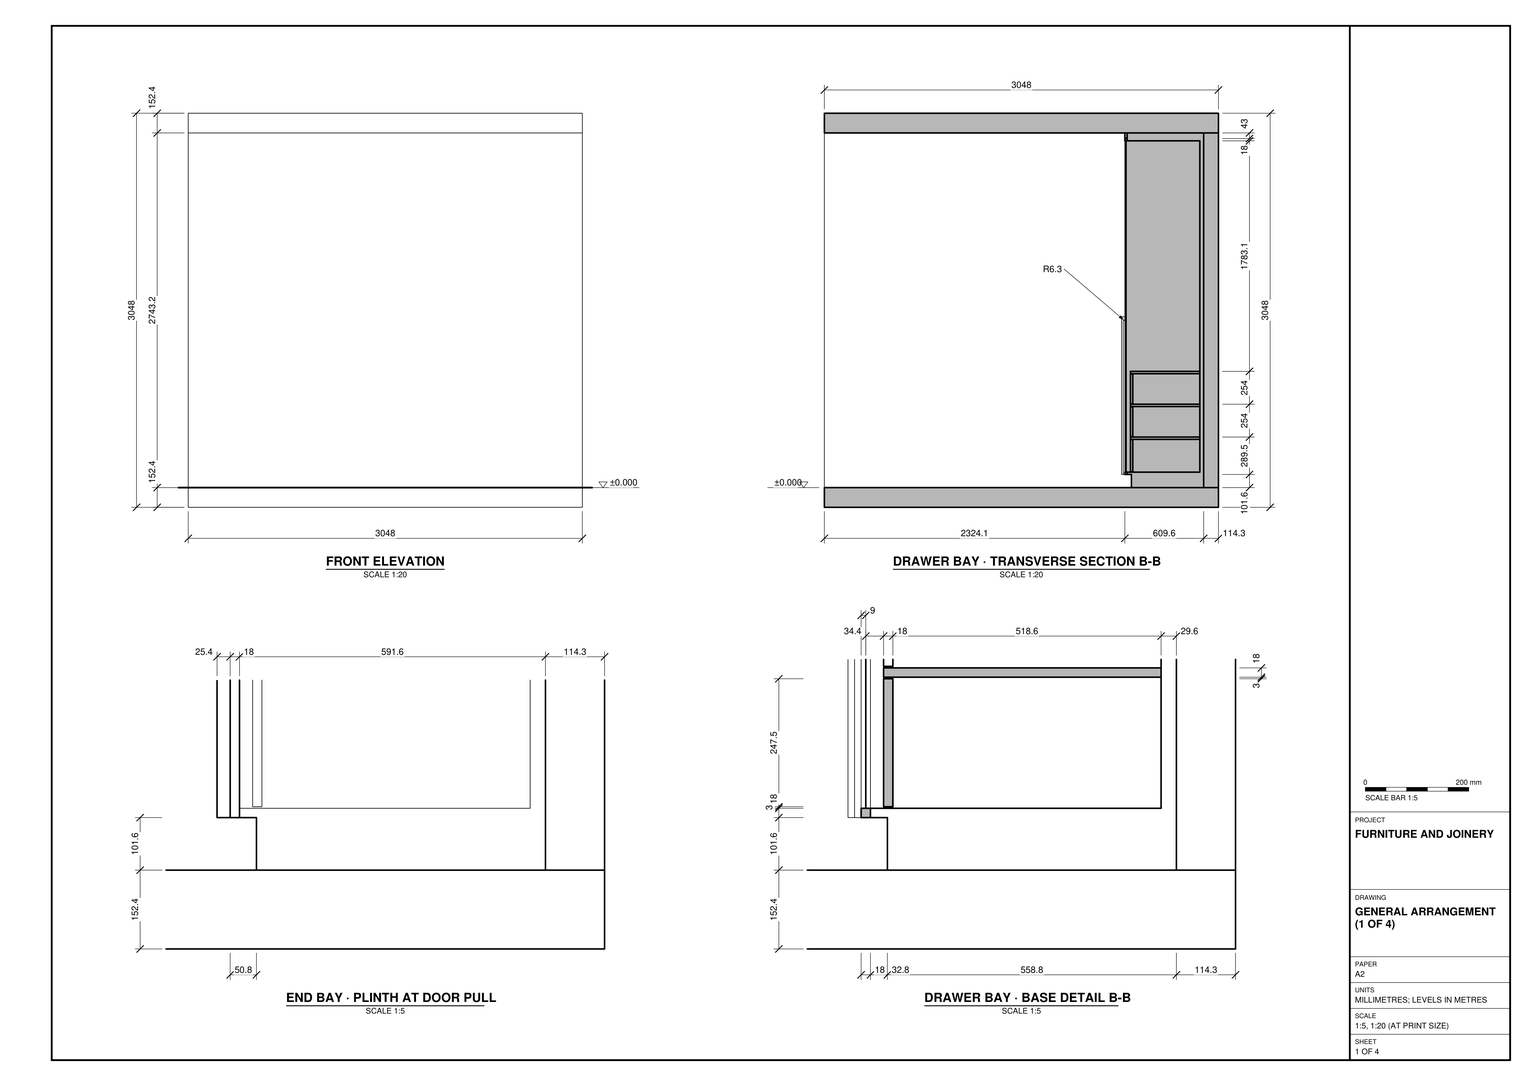
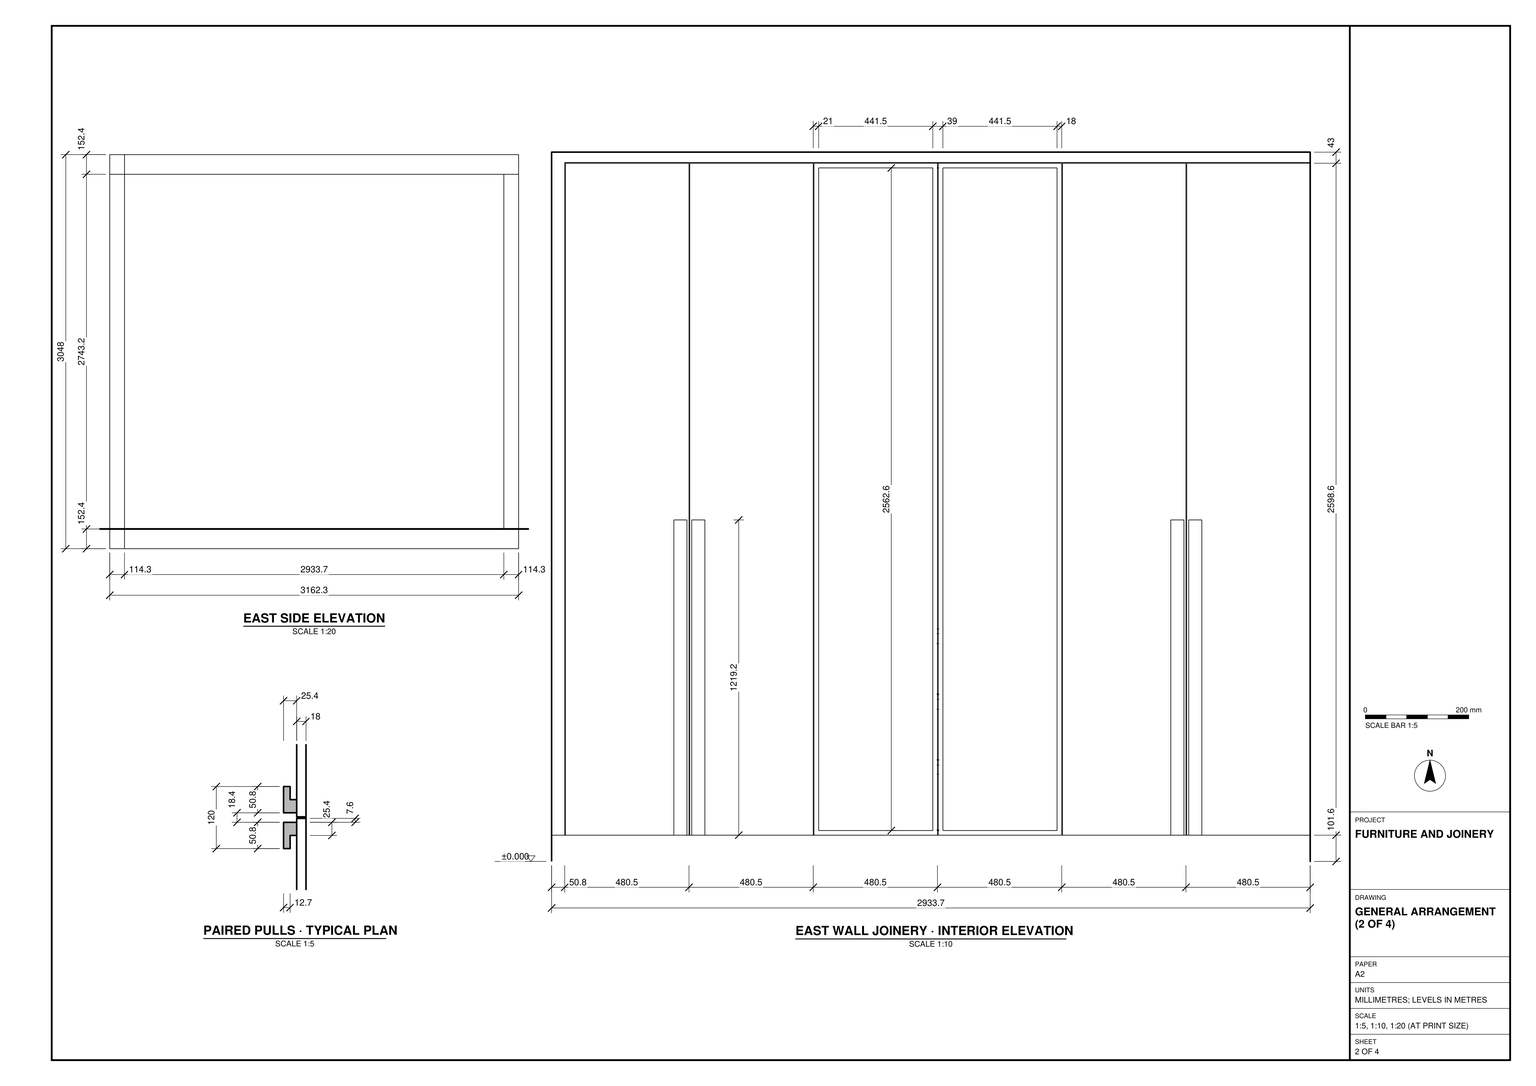
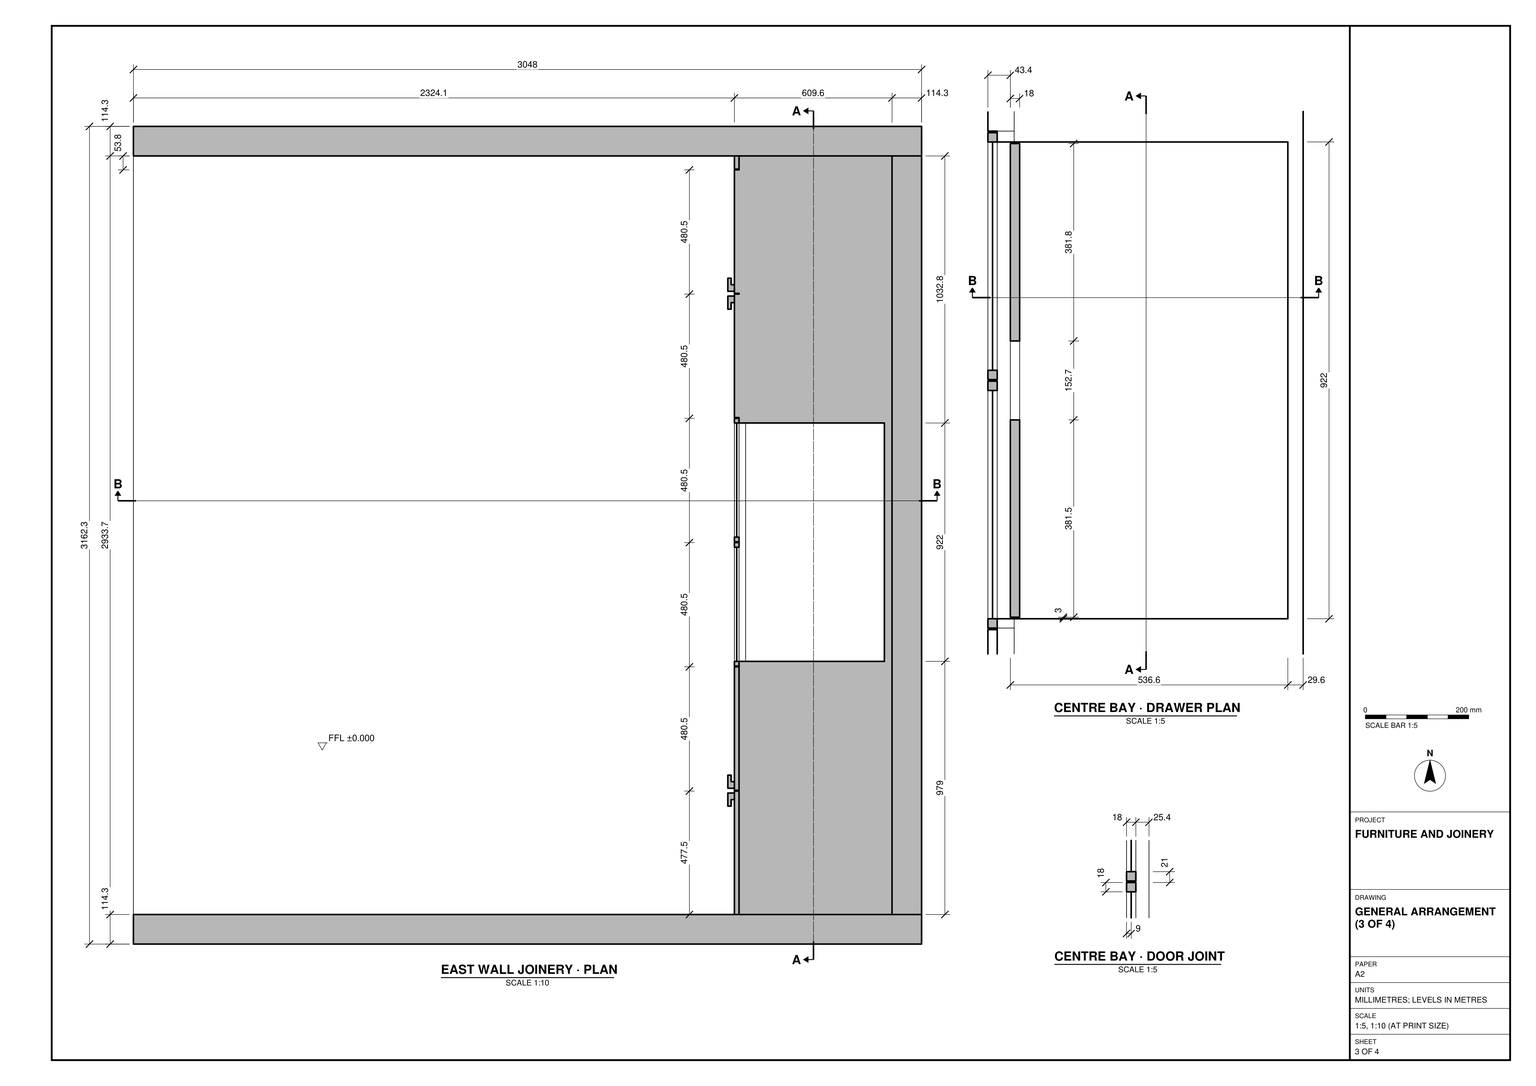
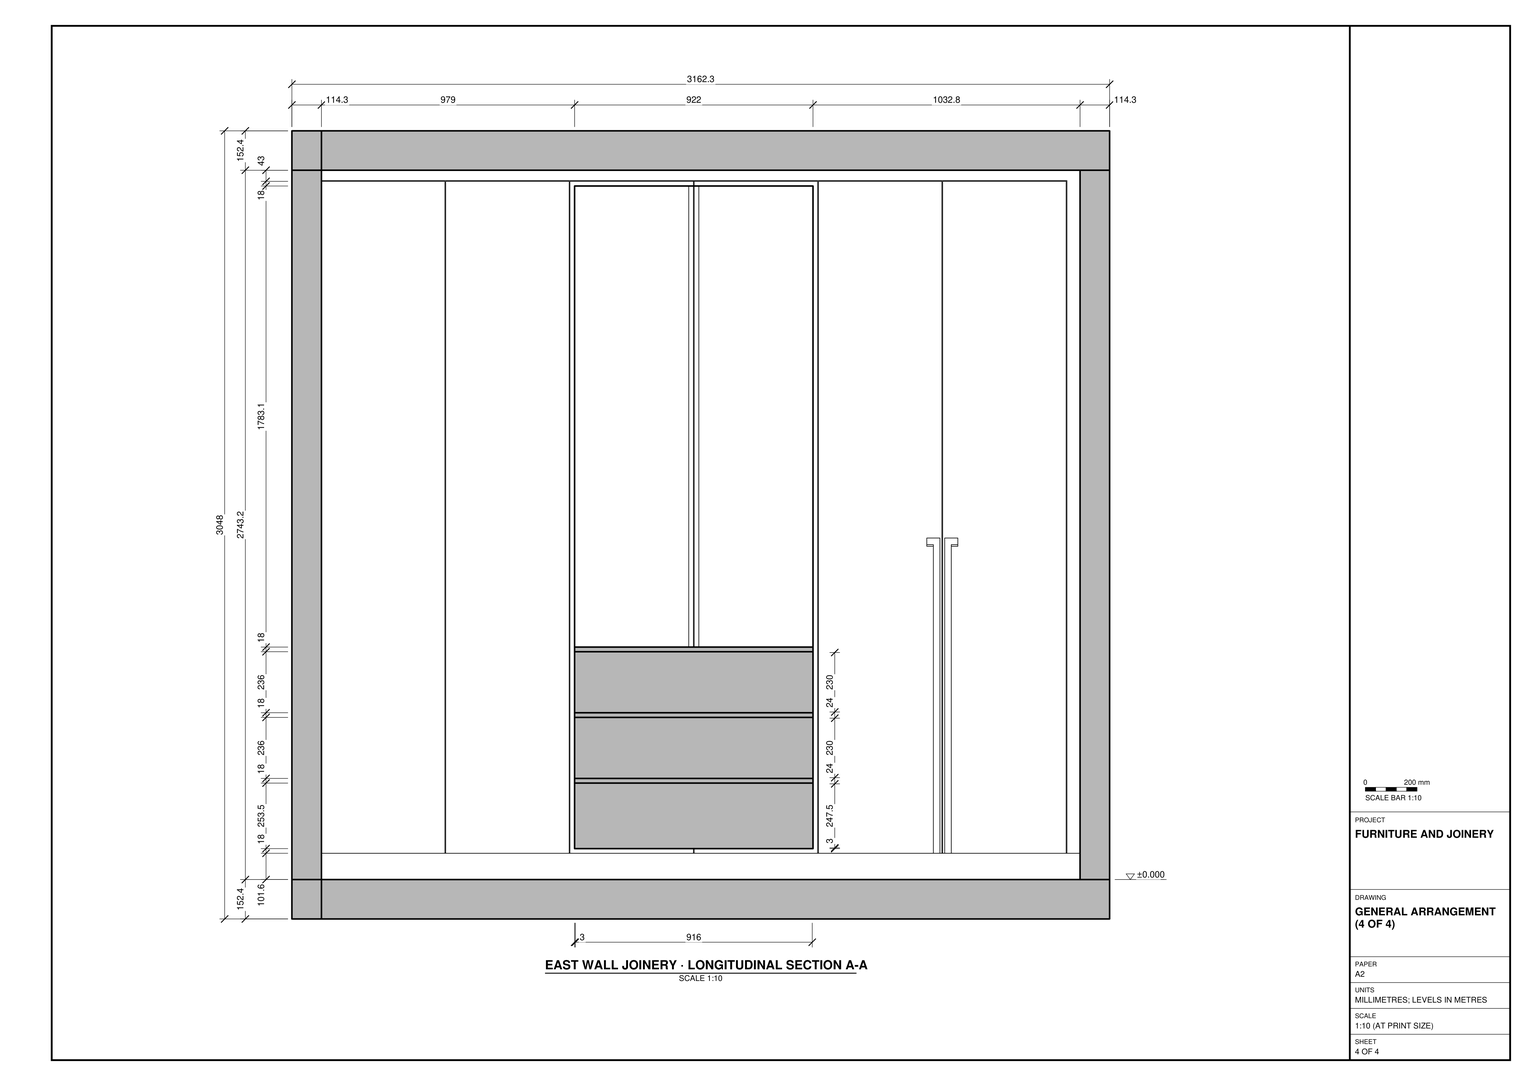
Work in millimetres in SketchUp from task_files/diagram_01.pdf. Model the full-height wardrobe along the east wall, together with the shell shown in plan and section. The overall extents are 3048 mm along X, 3162.3 mm along Y and 3048 mm vertically. Set the finished floor at the single storey level of 0 mm. Use the top of the floor slab, not its underside, as this datum. Model the floor and ceiling slabs and the east wall with its two return walls, leaving the opposite side open as drawn.

Fit the wardrobe between the return walls. Follow the interior elevation for the six tall fronts: the middle pair has narrow frames around inset panels, while the outer pairs have long vertical pulls at their meeting edges. Use the sections to set the cabinet depth, recess the plinth beneath the fronts and fit the narrow strip above them. Model the drawer stack low in the centre bay, leaving the space above it clear.

Keep the walls and slabs separate from one another and from the joinery. Organise the wardrobe and its distinct parts as groups or components, using components for repeated parts. Any decor or loose items may be suitable library components. Save one SketchUp model as output_files/east_wall_wardrobe_and_its_enclosing_shell.skp.

# SketchUp Ruby script. Lengths in millimetres.
U = 1.mm
M = Sketchup.active_model
def pt(a) = Geom::Point3d.new(a.map { |v| v * U })
def face(e, loops, mat)
  f = e.add_face(loops[0].map { |a| pt(a) })
  loops[1..].each { |l| e.add_face(l.map { |a| pt(a) }).erase! }
  f.material = f.back_material = mat if mat
  f
end
# faces: each face lists its corners as indices into pts; further lists are holes
def faces(e, pts, list, mat = nil) = list.each { |f| face(e, (f[0].is_a?(Array) ? f : [f]).map { |l| l.map { |i| pts[i] } }, mat) }
# xy, xz, yz: faces in a plane at the given z, y or x. An outline is a flat list of corners, or four numbers for a rectangle; further outlines are holes
def ring(l) = l.size == 4 ? [[l[0], l[1]], [l[2], l[1]], [l[2], l[3]], [l[0], l[3]]] : l.each_slice(2).to_a
def flat(e, list, mat, &to3) = list.each { |f| face(e, (f[0].is_a?(Array) ? f : [f]).map { |l| ring(l).map { |u, v| to3.(u, v) } }, mat) }
def xy(e, z, list, mat = nil) = flat(e, list, mat) { |x, y| [x, y, z] }
def xz(e, y, list, mat = nil) = flat(e, list, mat) { |x, z| [x, y, z] }
def yz(e, x, list, mat = nil) = flat(e, list, mat) { |y, z| [x, y, z] }
def lines(e, pts, list) = list.each { |a, b| e.add_line(pt(pts[a]), pt(pts[b])) }
# prism: a flat outline (further loops are holes) pulled along v
def prism(e, loops, v, mat = nil)
  f = face(e, loops, mat); d = Geom::Vector3d.new(v.map { |x| x * U })
  f.pushpull(f.normal.samedirection?(d) ? d.length : -d.length)
end
def box(e, o, s, mat = nil) = prism(e, [[o, [o[0] + s[0], o[1], o[2]], [o[0] + s[0], o[1] + s[1], o[2]], [o[0], o[1] + s[1], o[2]]]], [0, 0, s[2]], mat)
def at(x, y, z, deg = 0) = Geom::Transformation.translation(pt([x, y, z])) * Geom::Transformation.rotation(ORIGIN, Z_AXIS, deg.degrees)
def axes(o, x, y, z) = Geom::Transformation.new([*x, 0, *y, 0, *z, 0, *pt(o).to_a, 1])
def part(name) = M.definitions.add(name)
# library, detail: a bought-in or finely detailed component or shape, given as its bounding box
def library(name, o, s) = part(name).tap { |d| box(d.entities, o, s) }
def detail(e, o, s) = box(e.add_group.entities, o, s)
def put(e, d, t, mat = nil) = e.add_instance(d, t).tap { |i| i.material = mat if mat }
def group(e, t, mat = nil) = e.add_group.tap { |g| g.transformation = t; g.material = mat if mat }.entities
root = M.entities
M.materials.add("Tafisa-Mer-Calme-or-Calm-Sea-PM772-4K").color = [42, 58, 71]
M.materials.add("Tafisa-Rosee-du-Matin-or-Morning-Dew-PM763-4K").color = [198, 195, 187]
M.materials.add("[Color M09]").color = [0, 0, 0]
M.materials.add("[Translucent Glass Gray]").color = [128, 128, 128]
M.materials["[Translucent Glass Gray]"].alpha = 0.5
c1 = part("Group\#1")
xy(c1.entities,0,[[0,-114.3,3048,0],[0,0,3048,3048]])
xy(c1.entities,152.4,[[0,-114.3,3048,0],[0,0,3048,3048]])
xz(c1.entities,-114.3,[[0,0,3048,152.4]])
xz(c1.entities,0,[[0,0,3048,152.4]])
xz(c1.entities,3048,[[0,0,3048,152.4]])
yz(c1.entities,0,[[-114.3,0,0,152.4],[0,0,3048,152.4]])
yz(c1.entities,3048,[[-114.3,0,0,152.4],[0,0,3048,152.4]])
c2 = part("Group\#2")
box(c2.entities,[0,0,0],[3048,114.3,2743.2])
c3 = part("Group\#5")
box(c3.entities,[25.4,0,-18],[536.6,922,18])
c4 = part("Group\#9")
xy(c4.entities,0,[[0,0,0,50.8,25.4,50.8,25.4,25.4,12.7,25.4,12.7,0]])
xy(c4.entities,1219.2,[[0,0,25.4,50.8]])
xz(c4.entities,0,[[0,0,12.7,0,12.7,1187.2,12.9,1188.8,13.6,1190.4,14.6,1191.7,15.9,1192.7,17.4,1193.3,19,1193.6,20.7,1193.3,22.2,1192.7,23.5,1191.7,24.5,1190.4,25.2,1188.8,25.4,1187.2,25.4,1219.2,0,1219.2]])
xz(c4.entities,25.4,[[12.7,0,25.4,0,25.4,1187.2,25.2,1188.8,24.5,1190.4,23.5,1191.7,22.2,1192.7,20.7,1193.3,19,1193.6,17.4,1193.3,15.9,1192.7,14.6,1191.7,13.6,1190.4,12.9,1188.8,12.7,1187.2]])
xz(c4.entities,50.8,[[0,0,25.4,1219.2]])
yz(c4.entities,0,[[0,0,50.8,1219.2]])
yz(c4.entities,12.7,[[0,0,25.4,1187.2]])
yz(c4.entities,25.4,[[25.4,0,50.8,0,50.8,1219.2,0,1219.2,0,1187.2,25.4,1187.2]])
p = [[12.9,0,1188.8],[12.7,0,1187.2],[12.7,25.4,1187.2],[12.9,25.4,1188.8],[25.4,0,1187.2],[25.2,0,1188.8],
  [25.2,25.4,1188.8],[25.4,25.4,1187.2],[13.6,0,1190.4],[13.6,25.4,1190.4],[24.5,0,1190.4],[24.5,25.4,1190.4],
  [14.6,0,1191.7],[14.6,25.4,1191.7],[23.5,0,1191.7],[23.5,25.4,1191.7],[15.9,0,1192.7],[15.9,25.4,1192.7],
  [22.2,0,1192.7],[22.2,25.4,1192.7],[17.4,0,1193.3],[17.4,25.4,1193.3],[20.7,0,1193.3],[20.7,25.4,1193.3],
  [19,0,1193.6],[19,25.4,1193.6]]
faces(c4.entities,p,[[0,1,2,3],[4,5,6,7],[8,0,3,9],[5,10,11,6],[12,8,9,13],[10,14,15,11],[16,12,13,17],[14,18,19,15],
  [20,16,17,21],[18,22,23,19],[24,20,21,25],[22,24,25,23]])
yz(root,2333.1,[[1573.8,272,2015.2,2834.6]],"[Translucent Glass Gray]")
put(root,c1,at(0,114.3,0))
g1 = group(root,at(2933.7,114.3,152.4))
box(g1,[0,0,0],[114.3,2933.7,2743.2])
put(root,c2,at(0,3048,152.4))
g2 = group(root,at(2324.1,114.3,152.4),"Tafisa-Mer-Calme-or-Calm-Sea-PM772-4K")
xy(g2,0,[[50.8,0,609.6,2933.7]])
xy(g2,101.6,[[0,0,18,477.5],[18,0,50.8,961],[0,480.5,18,958],[18,961,50.8,1921.9],[0,1921.9,0,2399.4,18,2399.4,18,2402.4,0,2402.4,0,2879.9,18,2879.9,18,2882.9,50.8,2882.9,50.8,1921.9],
  [0,2882.9,18,2933.7],[18,2882.9,50.8,2933.7]])
xy(g2,101.6,[[0,961,18,1438.4],[0,1441.4,18,1918.9]],"[Color M09]")
xy(g2,119.6,[[18,979,580,1900.9]],"Tafisa-Rosee-du-Matin-or-Morning-Dew-PM763-4K")
xy(g2,119.6,[[0,979,9,1420.4],[9,979,18,1420.4],[0,1459.4,18,1900.9]],"[Color M09]")
xy(g2,2682.2,[[18,979,580,1900.9]],"Tafisa-Rosee-du-Matin-or-Morning-Dew-PM763-4K")
xy(g2,2682.2,[[0,979,9,1420.4],[9,979,18,1420.4],[0,1459.4,18,1900.9]],"[Color M09]")
xy(g2,2700.2,[[0,0,18,477.5],[0,480.5,18,958],[0,1921.9,18,2399.4],[0,2402.4,18,2879.9]])
xy(g2,2700.2,[[0,961,18,1438.5],[0,1441.5,18,1918.9]],"[Color M09]")
xy(g2,2703.2,[[0,0,18,2882.9]])
xy(g2,2743.2,[[0,0,18,2933.7],[18,0,609.6,2933.7]])
xz(g2,0,[[50.8,0,609.6,0,609.6,2743.2,18,2743.2,18,101.6,50.8,101.6],[0,101.6,18,2700.2],[0,2703.2,18,2743.2]])
xz(g2,477.5,[[0,101.6,18,2700.2]])
xz(g2,480.5,[[0,101.6,18,2700.2]])
xz(g2,958,[[0,101.6,18,2700.2]])
xz(g2,961,[[0,101.6,18,2700.2]])
xz(g2,979,[[18,119.6,580,2682.2]],"Tafisa-Rosee-du-Matin-or-Morning-Dew-PM763-4K")
xz(g2,979,[[0,119.6,9,2682.2],[9,119.6,18,2682.2]],"[Color M09]")
xz(g2,1420.4,[[0,119.6,9,2682.2],[9,119.6,18,2682.2]],"[Color M09]")
xz(g2,1459.4,[[0,119.6,18,2682.2]],"[Color M09]")
xz(g2,1900.9,[[18,119.6,580,2682.2]],"Tafisa-Rosee-du-Matin-or-Morning-Dew-PM763-4K")
xz(g2,1900.9,[[0,119.6,18,2682.2]],"[Color M09]")
xz(g2,1918.9,[[0,101.6,18,2700.2]],"[Color M09]")
xz(g2,1921.9,[[0,101.6,18,2700.2]])
xz(g2,2399.4,[[0,101.6,18,2700.2]])
xz(g2,2402.4,[[0,101.6,18,2700.2]])
xz(g2,2879.9,[[0,101.6,18,2700.2]])
xz(g2,2882.9,[[0,101.6,18,2703.2]])
xz(g2,2933.7,[[50.8,0,50.8,101.6,18,101.6,18,2743.2,609.6,2743.2,609.6,0],[0,101.6,18,2743.2]])
yz(g2,0,[[0,101.6,477.5,2700.2],[2882.9,101.6,2882.9,2703.2,0,2703.2,0,2743.2,2933.7,2743.2,2933.7,101.6],[480.5,101.6,958,2700.2],[1921.9,101.6,2399.4,2700.2],[2402.4,101.6,2879.9,2700.2]])
yz(g2,0,[[[961,101.6,961,2700.2,1438.5,2700.2,1438.4,101.6],[979,119.6,1420.4,2682.2]],[[1441.4,101.6,1441.5,2700.2,1918.9,2700.2,1918.9,101.6],[1459.4,119.6,1900.9,2682.2]]],"[Color M09]")
yz(g2,9,[[979,119.6,1420.4,2682.2]],"[Translucent Glass Gray]")
yz(g2,18,[[0,101.6,477.5,2700.2],[2882.9,101.6,2933.7,101.6,2933.7,2743.2,0,2743.2,0,2703.2,2882.9,2703.2],[477.5,101.6,477.5,2700.2,0,2700.2,0,2703.2,2882.9,2703.2,2882.9,101.6,2879.9,101.6,2879.9,2700.2,2402.4,2700.2,2402.4,101.6,2399.4,101.6,2399.4,2700.2,1921.9,2700.2,1921.9,101.6,1918.9,101.6,1918.9,2700.2,961,2700.2,961,101.6,958,101.6,958,2700.2,480.5,2700.2,480.5,101.6],[480.5,101.6,958,2700.2],[961,101.6,1438.4,101.6,1438.4,119.6,979,119.6,979,2682.2,1438.4,2682.2,1438.5,2700.2,961,2700.2],
  [1438.4,101.6,1441.4,119.6],[1441.4,101.6,1918.9,101.6,1918.9,2700.2,1441.5,2700.2,1441.4,2682.2,1900.9,2682.2,1900.9,119.6,1441.4,119.6],[1420.4,119.6,1438.4,2682.2],[1441.4,119.6,1459.4,2682.2],[1438.4,2682.2,1438.5,2700.2,1441.5,2700.2,1441.4,2682.2]])
yz(g2,50.8,[[0,0,2933.7,101.6]])
yz(g2,580,[[979,119.6,1900.9,2682.2]],"Tafisa-Rosee-du-Matin-or-Morning-Dew-PM763-4K")
yz(g2,609.6,[[0,0,2933.7,2743.2]])
p = [[0,1438.4,101.6],[0,1438.5,2700.2],[18,1438.5,2700.2],[18,1438.4,2682.2],[18,1438.4,119.6],[18,1438.4,101.6],
  [18,1441.4,101.6],[18,1441.4,119.6],[18,1441.4,2682.2],[18,1441.5,2700.2],[0,1441.5,2700.2],[0,1441.4,101.6]]
faces(g2,p,[[0,1,2,3,4,5],[6,7,8,9,10,11]],"[Color M09]")
put(g2,c3,at(18,979,391.1),"Tafisa-Rosee-du-Matin-or-Morning-Dew-PM763-4K")
put(g2,c3,at(18,979,645.1),"Tafisa-Rosee-du-Matin-or-Morning-Dew-PM763-4K")
put(g2,c3,at(18,979,899.1),"Tafisa-Rosee-du-Matin-or-Morning-Dew-PM763-4K")
g3 = group(root,at(2367.5,1093.3,797.5),"Tafisa-Rosee-du-Matin-or-Morning-Dew-PM763-4K")
prism(g3,[[[0,3,233],[0,384.8,233],[0,384.8,232.9],[0,385.8,222.1],[0,388.7,213.2],[0,393.6,206.3],[0,400.5,201.4],[0,409.4,198.4],[0,420.2,197.4],[0,501.7,197.4],[0,512.6,198.4],[0,521.4,201.4],[0,528.3,206.3],[0,533.2,213.2],[0,536.2,222.1],[0,537.2,232.9],[0,537.2,233],[0,919,233],[0,919,3],[0,3,3]]],[18,0,0])
g4 = group(root,at(2367.5,1093.3,543.5),"Tafisa-Rosee-du-Matin-or-Morning-Dew-PM763-4K")
prism(g4,[[[0,3,233],[0,384.8,233],[0,385.8,222.1],[0,388.8,213.2],[0,393.7,206.3],[0,400.7,201.4],[0,409.7,198.4],[0,420.6,197.4],[0,501.4,197.4],[0,512.3,198.4],[0,521.3,201.4],[0,528.2,206.3],[0,533.2,213.2],[0,536.2,222.1],[0,537.2,233],[0,919,233],[0,919,3],[0,3,3]]],[18,0,0])
g5 = group(root,at(2367.5,1093.3,289.5),"Tafisa-Rosee-du-Matin-or-Morning-Dew-PM763-4K")
prism(g5,[[[0,3,233],[0,384.5,233],[0,385.4,223.1],[0,388.1,214.9],[0,392.7,208.6],[0,399,204.1],[0,407.2,201.3],[0,417.2,200.4],[0,504.5,200.4],[0,514.5,201.3],[0,522.7,204.1],[0,529,208.6],[0,533.6,214.9],[0,536.3,223.1],[0,537.2,233],[0,919,233],[0,919,-14.5],[0,3,-14.5]]],[18,0,0])
put(root,c4,at(2298.7,533.4,254),"[Color M09]")
put(root,c4,axes([2298.7,653.4,254],[1,0,0],[0,-1,0],[0,0,1]),"[Color M09]")
put(root,c4,axes([2298.7,2575.3,254],[1,0,0],[0,-1,0],[0,0,1]),"[Color M09]")
put(root,c4,at(2298.7,2455.3,254),"[Color M09]")
put(root,c2,at(0,0,152.4))
put(root,c1,at(0,114.3,2895.6))
